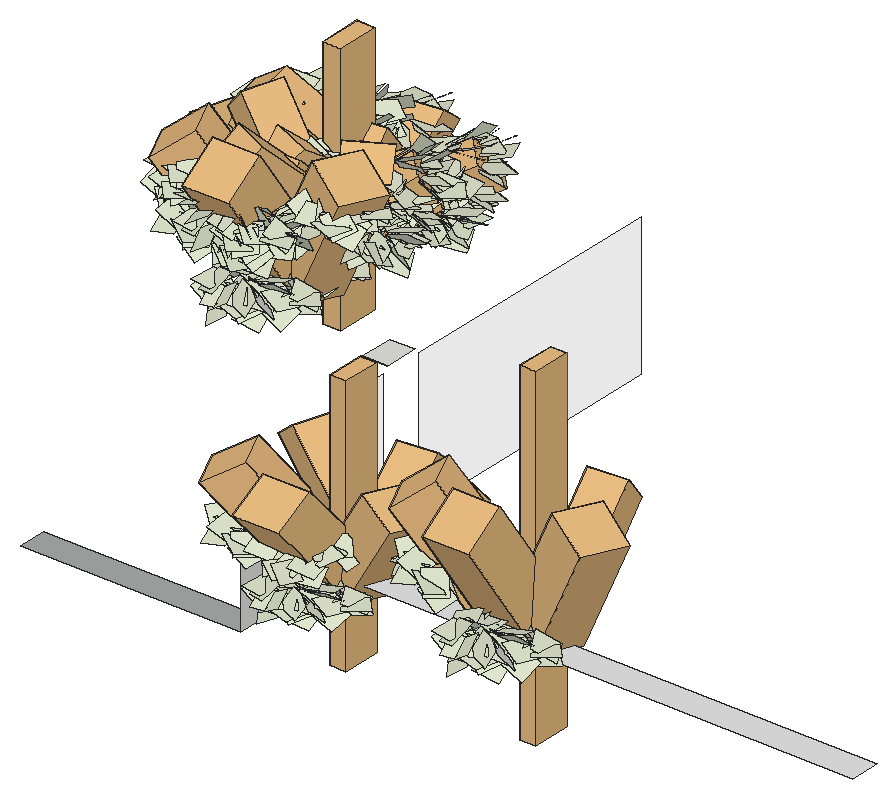
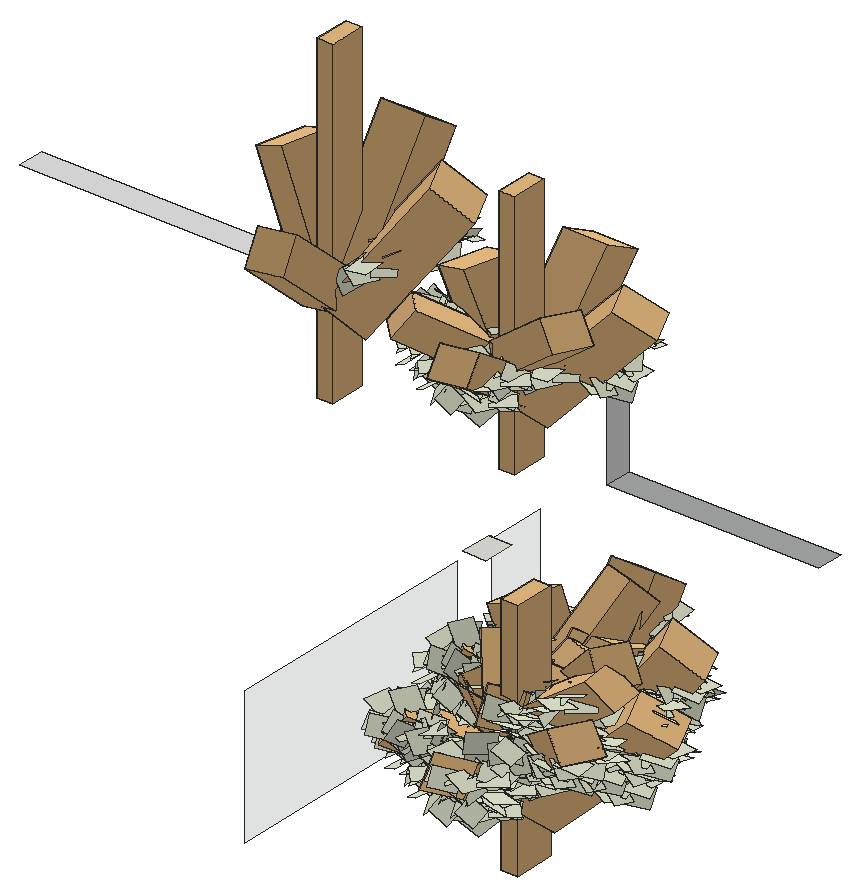
# SketchUp Ruby script. Lengths in inches.
U = 1.inch
M = Sketchup.active_model
def pt(a) = Geom::Point3d.new(a.map { |v| v * U })
def face(e, loops, mat)
  f = e.add_face(loops[0].map { |a| pt(a) })
  loops[1..].each { |l| e.add_face(l.map { |a| pt(a) }).erase! }
  f.material = f.back_material = mat if mat
  f
end
# faces: each face lists its corners as indices into pts; further lists are holes
def faces(e, pts, list, mat = nil) = list.each { |f| face(e, (f[0].is_a?(Array) ? f : [f]).map { |l| l.map { |i| pts[i] } }, mat) }
# xy, xz, yz: faces in a plane at the given z, y or x. An outline is a flat list of corners, or four numbers for a rectangle; further outlines are holes
def ring(l) = l.size == 4 ? [[l[0], l[1]], [l[2], l[1]], [l[2], l[3]], [l[0], l[3]]] : l.each_slice(2).to_a
def flat(e, list, mat, &to3) = list.each { |f| face(e, (f[0].is_a?(Array) ? f : [f]).map { |l| ring(l).map { |u, v| to3.(u, v) } }, mat) }
def xy(e, z, list, mat = nil) = flat(e, list, mat) { |x, y| [x, y, z] }
def xz(e, y, list, mat = nil) = flat(e, list, mat) { |x, z| [x, y, z] }
def yz(e, x, list, mat = nil) = flat(e, list, mat) { |y, z| [x, y, z] }
def lines(e, pts, list) = list.each { |a, b| e.add_line(pt(pts[a]), pt(pts[b])) }
# prism: a flat outline (further loops are holes) pulled along v
def prism(e, loops, v, mat = nil)
  f = face(e, loops, mat); d = Geom::Vector3d.new(v.map { |x| x * U })
  f.pushpull(f.normal.samedirection?(d) ? d.length : -d.length)
end
def box(e, o, s, mat = nil) = prism(e, [[o, [o[0] + s[0], o[1], o[2]], [o[0] + s[0], o[1] + s[1], o[2]], [o[0], o[1] + s[1], o[2]]]], [0, 0, s[2]], mat)
def at(x, y, z, deg = 0) = Geom::Transformation.translation(pt([x, y, z])) * Geom::Transformation.rotation(ORIGIN, Z_AXIS, deg.degrees)
def axes(o, x, y, z) = Geom::Transformation.new([*x, 0, *y, 0, *z, 0, *pt(o).to_a, 1])
def part(name) = M.definitions.add(name)
# library, detail: a bought-in or finely detailed component or shape, given as its bounding box
def library(name, o, s) = part(name).tap { |d| box(d.entities, o, s) }
def detail(e, o, s) = box(e.add_group.entities, o, s)
def put(e, d, t, mat = nil) = e.add_instance(d, t).tap { |i| i.material = mat if mat }
def group(e, t, mat = nil) = e.add_group.tap { |g| g.transformation = t; g.material = mat if mat }.entities
root = M.entities
M.materials.add("Celtis_australis_s cópia1").color = [224, 229, 205]
M.materials.add("[Concrete Form 4x8]").color = [167, 170, 168]
M.materials.add("[CoolGray4]").color = [225, 226, 230]
M.materials["[CoolGray4]"].alpha = 0.26
M.materials.add("[Polished Concrete Old]").color = [229, 229, 229]
M.materials.add("bark_cherry").color = [99, 76, 62]
c1 = library("trunk\#1",[0,0,0],[11.46,27.17,238.43])
c2 = part("branch2\#1")
p = [[13.74,0.36,0.5],[11.5,11.3125,10.98],[14.125,0.95,0],[14.97,0.95,0.19],[12.12,10.6875,11.67],[15.1,0.36,0.82],
  [11.05,10.4375,11.49],[14.34,0,1.01],[6.08,18.54,23.51],[6.83,18.32,23.89],[6.09,17.93,24.13],[3.27,29.37,34],
  [3.27,29.68,33.56],[3.73,29.59,33.82],[0,43.16,40.74],[0,43.16,40.75],[0.01,43.16,40.75],[5.59,23.2,32.77],
  [4.65,30.48,39.08],[1.92,39.79,43.02],[5.09,28.47,41.41]]
faces(c2.entities,p,[[0,1,2],[2,1,3],[3,4,5],[3,1,4],[6,0,7],[0,6,1],[5,6,7],[6,5,4],
  [6,8,1],[1,9,4],[9,1,8],[8,6,10],[4,10,6],[10,4,9],[10,11,8],[8,12,9],
  [12,8,11],[10,9,11],[13,11,9],[13,9,12],[14,12,11,15],[12,14,16,13],[13,16,15,11]],"bark_cherry")
lines(c2.entities,p,[[17,18],[11,19],[20,17],[17,10]])
c3 = library("branch1\#2",[0,0,0],[33.4,33.29,108.01])
c4 = part("leaf1\#1")
p = [[1.6,6.78,0.04],[-9.34,-4.04,0.02],[2.67,-16.2,2.05],[13.62,-5.38,2.07]]
faces(c4.entities,p,[[0,1,2,3]],"Celtis_australis_s cópia1")
c5 = part("leaf_group1\#1")
put(c5.entities,c4,axes([-0.06,3.68,7.3125],[0.53029,-0.80282,-0.27253],[0.82812,0.42159,0.36943],[-0.18168,-0.42159,0.8884]))
put(c5.entities,c4,axes([6.4375,-3.58,5.23],[1,0,0],[0,0.98927,0.14608],[0,-0.14608,0.98927]))
put(c5.entities,c4,axes([-0.99,3.68,1.22],[0.57591,-0.80282,0.15431],[0.36532,0.42159,0.82994],[-0.73135,-0.42159,0.53609]))
put(c5.entities,c4,axes([18.71,8.59,4.39],[0.33053,0.77491,0.53877],[-0.79988,-0.073,0.5957],[0.50094,-0.62785,0.5957]))
put(c5.entities,c4,axes([13.16,0.76,0.89],[0.89618,0.3501,0.27256],[-0.44248,0.65988,0.60727],[0.03275,-0.66482,0.74628]))
put(c5.entities,c4,axes([4.53,7.98,7.3125],[-0.1927,0.94265,-0.27253],[0.88368,0.28746,0.36943],[-0.42658,0.16964,0.8884]))
put(c5.entities,c4,axes([12.46,21.28,7.16],[0.85019,0.38493,0.35918],[0.30538,-0.91629,0.25914],[-0.42887,0.11063,0.89657]))
put(c5.entities,c4,axes([6.53,15.18,2.59],[0.70711,0.70711,0],[0.5,-0.5,0.70711],[-0.5,0.5,0.70711]))
put(c5.entities,c4,axes([-3.17,8.15,3.46],[-0.03719,0.74973,0.66069],[0.94096,-0.19634,0.27576],[-0.33647,-0.63194,0.69817]))
put(c5.entities,c4,axes([23.03,17.79,4.39],[0.78166,-0.31422,0.53877],[-0.61722,-0.51398,0.5957],[-0.08973,0.79818,0.5957]))
put(c5.entities,c4,axes([14.78,21.52,3.21],[0.67246,-0.04394,0.73882],[-0.28657,-0.93583,0.20517],[-0.6824,0.3497,0.64191]))
put(c5.entities,c4,axes([10.37,-1.8125,9],[0.99279,-0.06448,-0.101],[0.11527,0.74421,0.65792],[0.03275,-0.66482,0.74628]))
put(c5.entities,c4,axes([1.45,16.1875,2.9375],[-0.2106,-0.86579,-0.45394],[0.96054,-0.26957,0.06852],[-0.18168,-0.42159,0.8884]))
xy(root,40.75,[[506.24,57.05,645.65,75.24]],"[Concrete Form 4x8]")
xy(root,93.8125,[[645.65,57.05,1032.97,75.24]],"[Polished Concrete Old]")
xy(root,97.3125,[[582.23,233.07,597.61,254.44]])
xz(root,233.07,[[582.23,97.1875,597.61,97.3125]])
yz(root,597.61,[[189.81,2.93,230.14,94.26],[258.06,3.62,434.24,93.51]],"[CoolGray4]")
yz(root,645.65,[[57.05,40.75,75.24,93.8125]],"[Polished Concrete Old]")
put(root,c1,axes([453.91,361.34,14.57],[1,0,0],[0,1,0],[0,0,0.67]))
put(root,c1,axes([695.35,65.29,35.69],[0.89,0,0],[0,0.89,0],[0,0,0.6897]))
put(root,c1,axes([815.5,65.29,35.69],[0.89,0,0],[0,0.89,0],[0,0,0.89]))
put(root,c2,axes([453.37,328.85,55.76],[0.86505,0.20928,0],[0.18889,-0.78078,-0.38315],[0.0901,-0.37241,0.8033]))
put(root,c2,axes([444.22,374.54,56.54],[0.97196,0.23514,0],[0.21224,-0.87728,-0.28844],[0.10123,-0.41844,0.60473]))
put(root,c3,axes([441.04,340.06,44.32],[0.39386,-0.79787,0.01926],[0.63214,0.32498,0.53562],[-0.48721,-0.22335,0.71052]))
put(root,c5,axes([458.25,276.55,63.32],[0.7444,0.47059,-0.12848],[-0.47557,0.75228,0],[0.1086,0.06865,0.88068]))
put(root,c3,axes([430.37,387.14,47.93],[0.44254,-0.89649,0.0145],[0.71027,0.36515,0.40322],[-0.54743,-0.25096,0.53489]))
put(root,c5,axes([449.7,315.79,62.24],[0.83641,0.52876,-0.09672],[-0.53435,0.84526,0],[0.12202,0.07714,0.66298]))
put(root,c5,axes([486.91,288.45,67.29],[0.03841,0.87984,-0.12848],[-0.88915,0.03882,0],[0.0056,0.12835,0.88068]))
put(root,c5,axes([481.91,329.16,65.22],[0.04316,0.98858,-0.09672],[-0.99905,0.04362,0],[0.0063,0.14422,0.66298]))
put(root,c3,axes([478.68,345.14,53.8],[-0.69263,-0.11676,0.03129],[0.09962,-0.44829,0.53241],[-0.06847,0.52891,0.45816]))
put(root,c3,axes([479.16,306.41,57.15],[0.28975,0.83861,-0.06983],[-0.75053,0.29093,0.37969],[0.31209,-0.05308,0.65756]))
put(root,c3,axes([445.7,314.73,54.95],[0.89,0,0],[0,0.73347,0.5041],[0,-0.5041,0.73347]))
put(root,c3,axes([472.66,392.85,55.07],[-0.77824,-0.1312,0.02355],[0.11194,-0.5037,0.4008],[-0.07693,0.59428,0.34491]))
put(root,c5,axes([452.59,287.66,72.95],[0.53001,-0.70334,-0.12848],[0.71079,0.53562,0],[0.07732,-0.10261,0.88068]))
put(root,c3,axes([473.2,349.33,57.59],[0.32556,0.94226,-0.05257],[-0.84329,0.32689,0.28584],[0.35066,-0.05964,0.49502]))
put(root,c3,axes([435.61,358.68,55.93],[1,0,0],[0,0.82413,0.37949],[0,-0.56641,0.55216]))
put(root,c5,axes([443.34,328.27,69.48],[0.59551,-0.79027,-0.09672],[0.79864,0.60182,0],[0.08688,-0.11529,0.66298]))
put(root,c5,axes([424.58,362.36,83.74],[0.74616,0.33065,-0.38716],[-0.40514,0.91425,0],[0.52831,0.23411,0.54681]))
put(root,c5,axes([404.58,329.54,83.74],[0.74616,0.33065,-0.38716],[-0.40514,0.91425,0],[0.52831,0.23411,0.54681]))
put(root,c5,axes([435.89,318,91.88],[0.66408,0.29428,-0.51429],[-0.36058,0.81369,0],[0.47019,0.20836,0.72636]))
put(root,c5,axes([418.09,288.8,91.88],[0.66408,0.29428,-0.51429],[-0.36058,0.81369,0],[0.47019,0.20836,0.72636]))
put(root,c5,axes([441.11,435.57,75.26],[-0.04316,-0.98858,-0.09672],[0.99905,-0.04362,0],[-0.0063,-0.14422,0.66298]))
put(root,c5,axes([457.86,413.94,75.26],[-0.04316,-0.98858,-0.09672],[0.99905,-0.04362,0],[-0.0063,-0.14422,0.66298]))
put(root,c5,axes([450.6,383.16,80.62],[-0.03841,-0.87984,-0.12848],[0.88915,-0.03882,0],[-0.0056,-0.12835,0.88068]))
put(root,c5,axes([465.51,363.91,80.62],[-0.03841,-0.87984,-0.12848],[0.88915,-0.03882,0],[-0.0056,-0.12835,0.88068]))
put(root,c3,axes([477.09,374.68,63.34],[-0.55221,0.57381,0.05108],[-0.27657,-0.3541,0.44348],[0.45765,0.38748,0.267]))
put(root,c5,axes([396.35,362.32,73.7],[0.65426,-0.7553,-0.02572],[0.75585,0.65474,0],[0.02513,-0.02902,0.66951]))
put(root,c3,axes([482.625,328.97,64.79],[-0.49147,0.51069,0.06785],[-0.24614,-0.31515,0.5891],[0.40731,0.34486,0.35468]))
put(root,c5,axes([410.77,317.97,78.55],[0.58229,-0.67221,-0.03417],[0.67271,0.58272,0],[0.02237,-0.02582,0.88934]))
put(root,c2,axes([686.73,77.03,78.9],[0.86505,0.20928,0],[0.18889,-0.78078,-0.29692],[0.0901,-0.37241,0.62251]))
put(root,c5,axes([503.39,402.91,80.53],[-0.05351,0.98808,-0.09672],[-0.99854,-0.05408,0],[-0.00781,0.14414,0.66298]))
put(root,c5,axes([493.2,402.91,80.53],[-0.05351,0.98808,-0.09672],[-0.99854,-0.05408,0],[-0.00781,0.14414,0.66298]))
put(root,c5,axes([523.4,377.97,82.63],[-0.66851,0.72955,-0.09672],[-0.73728,-0.67559,0],[-0.09753,0.10643,0.66298]))
put(root,c5,axes([441.11,423.75,82.8],[-0.04316,-0.98858,-0.09672],[0.99905,-0.04362,0],[-0.0063,-0.14422,0.66298]))
put(root,c5,axes([506.03,354.09,87.63],[-0.04763,0.87939,-0.12848],[-0.8887,-0.04813,0],[-0.00695,0.12829,0.88068]))
put(root,c5,axes([496.96,354.09,87.63],[-0.04763,0.87939,-0.12848],[-0.8887,-0.04813,0],[-0.00695,0.12829,0.88068]))
put(root,c3,axes([674.4,88.25,70.04],[0.39386,-0.79787,0.01493],[0.63214,0.32498,0.41507],[-0.48721,-0.22335,0.55061]))
put(root,c5,axes([469.13,424.89,84.22],[0.04316,0.98858,-0.09672],[-0.99905,0.04362,0],[0.0063,0.14422,0.66298]))
put(root,c5,axes([691.61,24.74,84.76],[0.7444,0.47059,-0.09956],[-0.47557,0.75228,0],[0.1086,0.06865,0.68247]))
put(root,c5,axes([523.84,331.9,90.41],[-0.59498,0.6493,-0.12848],[-0.65618,-0.60128,0],[-0.0868,0.09472,0.88068]))
put(root,c5,axes([450.6,372.64,90.63],[-0.03841,-0.87984,-0.12848],[0.88915,-0.03882,0],[-0.0056,-0.12835,0.88068]))
put(root,c5,axes([468.75,323.39,85.98],[-0.46214,0.87795,0.08376],[-0.88678,-0.45652,-0.04836],[-0.0063,-0.14422,0.66298]))
put(root,c3,axes([453.65,402.0625,75.36],[-0.31066,-0.7342,-0.04462],[0.49665,-0.26184,0.38183],[-0.49034,0.16196,0.33616]))
put(root,c5,axes([495.37,378.48,87.32],[0.66851,-0.72955,-0.09672],[0.73728,0.67559,0],[0.09753,-0.10643,0.66298]))
put(root,c5,axes([720.27,36.64,87.84],[0.03841,0.87984,-0.09956],[-0.88915,0.03882,0],[0.0056,0.12835,0.68247]))
put(root,c5,axes([459.75,352.51,88.1],[0.98953,0,-0.09672],[0,1,0],[0.14436,0,0.66298]))
put(root,c5,axes([475.54,373.66,92.52],[0.03841,0.87984,-0.12848],[-0.88915,0.03882,0],[0.0056,0.12835,0.88068]))
put(root,c2,axes([806.88,77.03,91.45],[0.86505,0.20928,0],[0.18889,-0.78078,-0.38315],[0.0901,-0.37241,0.8033]))
put(root,c5,axes([397.71,340.85,88.6],[0.66774,0.73026,-0.09672],[-0.73799,0.67481,0],[0.09741,0.10653,0.66298]))
put(root,c5,axes([451.57,424.89,88.87],[0.04316,0.98858,-0.09672],[-0.99905,0.04362,0],[0.0063,0.14422,0.66298]))
put(root,c5,axes([496.92,418.82,88.91],[-0.04316,-0.98858,-0.09672],[0.99905,-0.04362,0],[-0.0063,-0.14422,0.66298]))
put(root,c5,axes([401.73,378.69,86.81],[0.65426,-0.7553,-0.02572],[0.75585,0.65474,0],[0.02513,-0.02902,0.66951]))
put(root,c5,axes([425.32,394.5625,90.2],[0.59551,-0.79027,-0.09672],[0.79864,0.60182,0],[0.08688,-0.11529,0.66298]))
put(root,c3,axes([712.04,93.33,77.39],[-0.69263,-0.11676,0.02425],[0.09962,-0.44829,0.41258],[-0.06847,0.52891,0.35505]))
put(root,c5,axes([475.2,283.32,94.86],[-0.41131,0.78137,0.11126],[-0.78924,-0.4063,-0.06424],[-0.0056,-0.12835,0.88068]))
put(root,c3,axes([712.52,54.59,79.98],[0.28975,0.83861,-0.05411],[-0.75053,0.29093,0.29424],[0.31209,-0.05308,0.50957]))
put(root,c3,axes([679.0625,62.92,78.27],[0.89,0,0],[0,0.73347,0.39065],[0,-0.5041,0.5684]))
put(root,c5,axes([489.31,427,97.52],[0.04393,-0.98858,-0.09656],[0.83213,-0.04362,0.37042],[-0.55284,-0.14422,0.54988]))
put(root,c5,axes([685.95,35.85,92.22],[0.53001,-0.70334,-0.09956],[0.71079,0.53562,0],[0.07732,-0.10261,0.68247]))
put(root,c3,axes([461.76,353.34,80.75],[-0.27649,-0.65344,-0.05927],[0.44202,-0.23304,0.50721],[-0.4364,0.14415,0.44654]))
put(root,c5,axes([473.82,314.55,95.67],[0.29786,0.92406,-0.16053],[-0.9435,0.32314,0.04914],[0.14519,0.20421,0.64863]))
put(root,c5,axes([434.82,323.22,95.67],[0.59551,-0.76679,-0.16053],[0.79864,0.59733,0.04914],[0.08688,-0.23502,0.64863]))
put(root,c5,axes([508.33,394.54,92.13],[-0.05351,0.98808,-0.09672],[-0.99854,-0.05408,0],[-0.00781,0.14414,0.66298]))
put(root,c5,axes([498.89,332.35,96.64],[0.59498,-0.6493,-0.12848],[0.65618,0.60128,0],[0.0868,-0.09472,0.88068]))
put(root,c5,axes([407.9,394.58,92.33],[0.59551,-0.79027,-0.09672],[0.79864,0.60182,0],[0.08688,-0.11529,0.66298]))
put(root,c3,axes([794.55,88.25,80.02],[0.39386,-0.79787,0.01926],[0.63214,0.32498,0.53562],[-0.48721,-0.22335,0.71052]))
put(root,c5,axes([467.19,309.24,97.68],[0.88068,0,-0.12848],[0,0.89,0],[0.12848,0,0.88068]))
put(root,c5,axes([437.21,392.42,97.71],[0.84181,0.51031,0.11785],[-0.46746,0.85217,-0.15755],[-0.2699,0.11572,0.64046]))
put(root,c5,axes([459.75,313.83,93.84],[0.98953,0,-0.09672],[0,1,0],[0.14436,0,0.66298]))
put(root,c5,axes([411.98,298.86,98.35],[0.59429,0.64993,-0.12848],[-0.65681,0.60058,0],[0.0867,0.09481,0.88068]))
put(root,c5,axes([459.91,373.66,98.7],[0.03841,0.87984,-0.12848],[-0.88915,0.03882,0],[0.0056,0.12835,0.88068]))
put(root,c5,axes([500.27,368.25,98.75],[-0.03841,-0.87984,-0.12848],[0.88915,-0.03882,0],[-0.0056,-0.12835,0.88068]))
put(root,c5,axes([811.76,24.74,99.02],[0.7444,0.47059,-0.12848],[-0.47557,0.75228,0],[0.1086,0.06865,0.88068]))
put(root,c5,axes([669.25,66.1875,106.89],[0.66408,0.29428,-0.39855],[-0.36058,0.81369,0],[0.47019,0.20836,0.56289]))
put(root,c5,axes([651.45,36.99,106.89],[0.66408,0.29428,-0.39855],[-0.36058,0.81369,0],[0.47019,0.20836,0.56289]))
put(root,c5,axes([415.55,332.54,95.96],[0.58229,-0.67221,-0.03417],[0.67271,0.58272,0],[0.02237,-0.02582,0.88934]))
put(root,c5,axes([381.81,362.85,95.76],[0.62273,-0.76901,-0.09672],[0.77715,0.62932,0],[0.09085,-0.11219,0.66298]))
put(root,c5,axes([399,335.5,95.76],[0.98953,0,-0.09672],[0,1,0],[0.14436,0,0.66298]))
put(root,c5,axes([436.55,346.67,100.46],[0.53001,-0.70334,-0.12848],[0.71079,0.53562,0],[0.07732,-0.10261,0.88068]))
put(root,c5,axes([434.82,320.57,100.89],[0.59551,-0.78385,0.11785],[0.79864,0.55397,-0.15755],[0.08688,0.28052,0.64046]))
put(root,c5,axes([441.11,445.07,97.12],[-0.04316,-0.98858,-0.09672],[0.99905,-0.04362,0],[-0.0063,-0.14422,0.66298]))
put(root,c5,axes([683.96,131.35,98.17],[-0.03841,-0.87984,-0.09956],[0.88915,-0.03882,0],[-0.0056,-0.12835,0.68247]))
put(root,c5,axes([698.87,112.1,98.17],[-0.03841,-0.87984,-0.09956],[0.88915,-0.03882,0],[-0.0056,-0.12835,0.68247]))
put(root,c5,axes([493.5,375.54,110.19],[0.0391,-0.87984,-0.12827],[0.74059,-0.03882,0.49205],[-0.49203,-0.12835,0.73043]))
put(root,c5,axes([840.42,36.64,102.98],[0.03841,0.87984,-0.12848],[-0.88915,0.03882,0],[0.0056,0.12835,0.88068]))
put(root,c5,axes([479.72,275.45,107.74],[0.26509,0.82241,-0.21324],[-0.83972,0.2876,0.06528],[0.12922,0.18175,0.86161]))
put(root,c5,axes([445,283.17,107.74],[0.53001,-0.68244,-0.21324],[0.71079,0.53162,0.06528],[0.07732,-0.20917,0.86161]))
put(root,c5,axes([510.42,346.64,103.04],[-0.04763,0.87939,-0.12848],[-0.8887,-0.04813,0],[-0.00695,0.12829,0.88068]))
put(root,c3,axes([469.33,361.6,85.43],[-0.7431,0.28874,0.04462],[0.24699,0.5042,0.38183],[-0.1223,-0.41079,0.27901]))
put(root,c5,axes([421.04,346.68,103.3],[0.53001,-0.70334,-0.12848],[0.71079,0.53562,0],[0.07732,-0.10261,0.88068]))
put(root,c3,axes([715.99,77.16,85.9],[-0.49147,0.51069,0.05258],[-0.24614,-0.31515,0.45652],[0.40731,0.34486,0.27485]))
put(root,c5,axes([644.125,66.16,96.57],[0.58229,-0.67221,-0.02648],[0.67271,0.58272,0],[0.02237,-0.02582,0.68919]))
put(root,c5,axes([495.14,343,99.5],[0.85173,0.50371,-0.09672],[-0.50904,0.86074,0],[0.12425,0.07348,0.66298]))
put(root,c5,axes([508.33,358.97,99.5],[-0.05351,0.98808,-0.09672],[-0.99854,-0.05408,0],[-0.00781,0.14414,0.66298]))
put(root,c5,axes([496.92,427,100.26],[-0.04316,-0.98858,-0.09672],[0.99905,-0.04362,0],[-0.0063,-0.14422,0.66298]))
put(root,c5,axes([447.13,344.76,110.4375],[0.74921,0.45418,0.15655],[-0.41604,0.75843,-0.20928],[-0.24021,0.10299,0.85076]))
put(root,c5,axes([467.19,274.8125,105.3],[0.88068,0,-0.12848],[0,0.89,0],[0.12848,0,0.88068]))
put(root,c5,axes([399,340.8125,101.25],[0.98953,0,-0.09672],[0,1,0],[0.14436,0,0.66298]))
put(root,c5,axes([415.68,382.08,102.42],[0.83641,0.52876,-0.09672],[-0.53435,0.84526,0],[0.12202,0.07714,0.66298]))
put(root,c3,axes([832.1875,93.33,89.49],[-0.69263,-0.11676,0.03129],[0.09962,-0.44829,0.53241],[-0.06847,0.52891,0.45816]))
put(root,c5,axes([739.39,102.28,103.6],[-0.04763,0.87939,-0.09956],[-0.8887,-0.04813,0],[-0.00695,0.12829,0.68247]))
put(root,c5,axes([730.32,102.28,103.6],[-0.04763,0.87939,-0.09956],[-0.8887,-0.04813,0],[-0.00695,0.12829,0.68247]))
put(root,c5,axes([434.82,346.34,106.8125],[0.59551,-0.76679,-0.16053],[0.79864,0.59733,0.04914],[0.08688,-0.23502,0.64863]))
put(root,c5,axes([459.03,299.73,107.63],[0.84181,0.51031,0.11785],[-0.46746,0.85217,-0.15755],[-0.2699,0.11572,0.64046]))
put(root,c3,axes([480.41,379.87,90.16],[-0.64428,-0.46954,0.04462],[-0.29101,0.48014,0.38183],[0.27972,-0.32475,0.27901]))
put(root,c5,axes([397.82,318.44,107.86],[0.55423,-0.68442,-0.12848],[0.69166,0.5601,0],[0.08085,-0.09985,0.88068]))
put(root,c5,axes([413.125,294.1,107.86],[0.88068,0,-0.12848],[0,0.89,0],[0.12848,0,0.88068]))
put(root,c5,axes([437.21,392.42,108.05],[0.84181,0.51031,0.11785],[-0.46746,0.85217,-0.15755],[-0.2699,0.11572,0.64046]))
put(root,c3,axes([832.67,54.59,92.84],[0.28975,0.83861,-0.06983],[-0.75053,0.29093,0.37969],[0.31209,-0.05308,0.65756]))
put(root,c3,axes([799.21,62.92,90.64],[0.89,0,0],[0,0.73347,0.5041],[0,-0.5041,0.73347]))
put(root,c5,axes([806.1,35.85,108.64],[0.53001,-0.70334,-0.12848],[0.71079,0.53562,0],[0.07732,-0.10261,0.88068]))
put(root,c5,axes([445,280.8125,114.67],[0.53001,-0.69763,0.15655],[0.71079,0.49304,-0.20928],[0.07732,0.24966,0.85076]))
put(root,c5,axes([450.6,391.61,109.66],[-0.03841,-0.87984,-0.12848],[0.88915,-0.03882,0],[-0.0056,-0.12835,0.88068]))
put(root,c5,axes([757.2,80.09,105.75],[-0.59498,0.6493,-0.09956],[-0.65618,-0.60128,0],[-0.0868,0.09472,0.68247]))
put(root,c5,axes([683.96,120.83,105.93],[-0.03841,-0.87984,-0.09956],[0.88915,-0.03882,0],[-0.0056,-0.12835,0.68247]))
put(root,c5,axes([418.99,380.5,127.125],[0.3711,-0.79027,-0.32669],[0.61978,0.60182,-0.33747],[0.69149,-0.11529,0.4778]))
put(root,c5,axes([401.55,382.08,106.19],[0.83641,0.52876,-0.09672],[-0.53435,0.84526,0],[0.12202,0.07714,0.66298]))
put(root,c5,axes([488.3,361.44,106.29],[-0.04316,-0.98858,-0.09672],[0.99905,-0.04362,0],[-0.0063,-0.14422,0.66298]))
put(root,c5,axes([708.9,121.84,107.39],[0.03841,0.87984,-0.09956],[-0.88915,0.03882,0],[0.0056,0.12835,0.68247]))
put(root,c3,axes([475.72,317.33,94.125],[-0.66136,0.25698,0.05927],[0.21982,0.44874,0.50721],[-0.10884,-0.3656,0.37063]))
put(root,c5,axes([434.82,343.7,112.03],[0.59551,-0.78385,0.11785],[0.79864,0.55397,-0.15755],[0.08688,0.28052,0.64046]))
put(root,c5,axes([516.32,362.58,107.71],[0.04316,0.98858,-0.09672],[-0.99905,0.04362,0],[0.0063,0.14422,0.66298]))
put(root,c3,axes([447.15,363.93,94.89],[-0.13796,0.78519,0.04462],[0.55922,0.04992,0.38183],[-0.41473,-0.10819,0.27901]))
put(root,c5,axes([510.42,314.99,112.83],[-0.04763,0.87939,-0.12848],[-0.8887,-0.04813,0],[-0.00695,0.12829,0.88068]))
put(root,c5,axes([498.69,300.77,112.83],[0.75804,0.4483,-0.12848],[-0.45305,0.76606,0],[0.11059,0.0654,0.88068]))
put(root,c5,axes([789.4,66.1875,127.57],[0.66408,0.29428,-0.51429],[-0.36058,0.81369,0],[0.47019,0.20836,0.72636]))
put(root,c5,axes([771.6,36.99,127.57],[0.66408,0.29428,-0.51429],[-0.36058,0.81369,0],[0.47019,0.20836,0.72636]))
put(root,c5,axes([459.75,313.83,108.87],[0.98953,0,-0.09672],[0,1,0],[0.14436,0,0.66298]))
put(root,c5,axes([399,335.5,108.87],[0.98953,0,-0.09672],[0,1,0],[0.14436,0,0.66298]))
put(root,c5,axes([708.57,31.51,109.21],[-0.41131,0.78137,0.08622],[-0.78924,-0.4063,-0.04978],[-0.0056,-0.12835,0.68247]))
put(root,c5,axes([500.27,375.54,113.83],[-0.03841,-0.87984,-0.12848],[0.88915,-0.03882,0],[-0.0056,-0.12835,0.88068]))
put(root,c3,axes([695.12,101.53,98.27],[-0.27649,-0.65344,-0.04593],[0.44202,-0.23304,0.39305],[-0.4364,0.14415,0.34604]))
put(root,c5,axes([732.25,80.54,110.58],[0.59498,-0.6493,-0.09956],[0.65618,0.60128,0],[0.0868,-0.09472,0.68247]))
put(root,c5,axes([413.125,298.83,115.15],[0.88068,0,-0.12848],[0,0.89,0],[0.12848,0,0.88068]))
put(root,c5,axes([700.55,57.43,111.39],[0.88068,0,-0.09956],[0,0.89,0],[0.12848,0,0.68247]))
